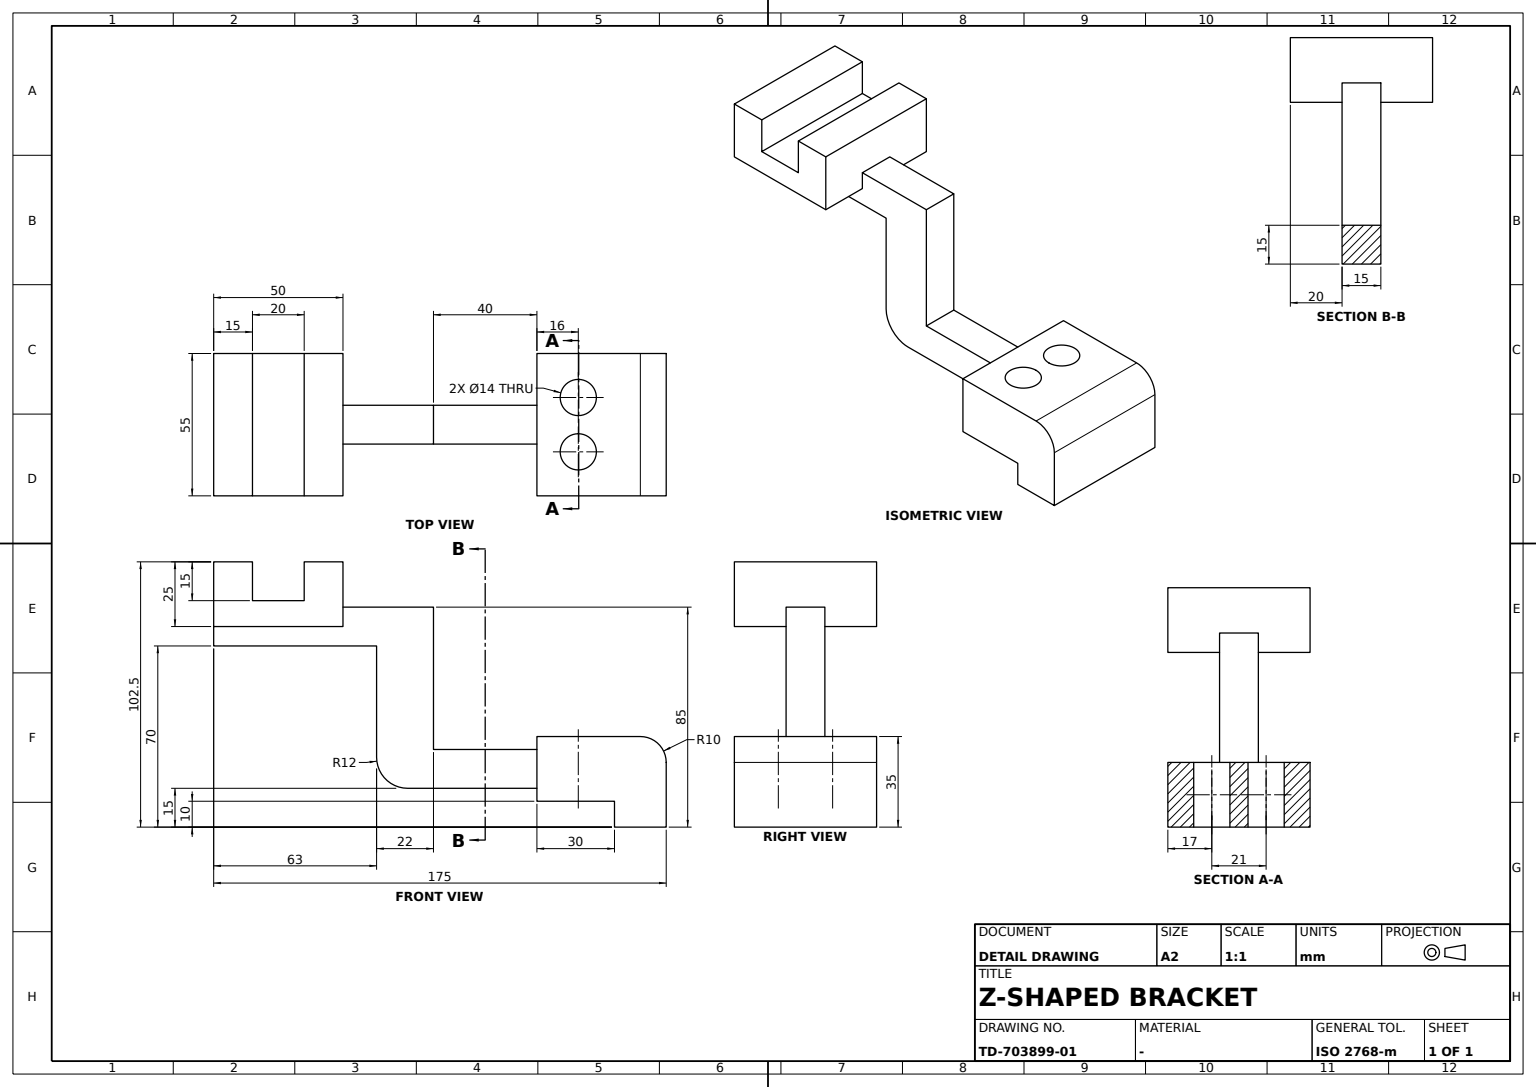
ISO-10303-21;
HEADER;
FILE_DESCRIPTION((''),'2;1');
FILE_NAME('','',(''),(''),'','','');
FILE_SCHEMA(('AUTOMOTIVE_DESIGN'));
ENDSEC;
DATA;
#1=APPLICATION_CONTEXT('');
#2=PRODUCT_CONTEXT('',#1,'mechanical');
#3=PRODUCT('','','',(#2));
#4=PRODUCT_DEFINITION_FORMATION('','',#3);
#5=PRODUCT_DEFINITION_CONTEXT('',#1,'design');
#6=PRODUCT_DEFINITION('','',#4,#5);
#7=PRODUCT_DEFINITION_SHAPE('','',#6);
#8=(LENGTH_UNIT()NAMED_UNIT(*)SI_UNIT(.MILLI.,.METRE.));
#9=(NAMED_UNIT(*)PLANE_ANGLE_UNIT()SI_UNIT($,.RADIAN.));
#10=(NAMED_UNIT(*)SI_UNIT($,.STERADIAN.)SOLID_ANGLE_UNIT());
#11=UNCERTAINTY_MEASURE_WITH_UNIT(LENGTH_MEASURE(0.005),#8,'distance_accuracy_value','');
#12=(GEOMETRIC_REPRESENTATION_CONTEXT(3)GLOBAL_UNCERTAINTY_ASSIGNED_CONTEXT((#11))GLOBAL_UNIT_ASSIGNED_CONTEXT((#8,#9,#10))REPRESENTATION_CONTEXT('',''));
#13=CARTESIAN_POINT('',(-17.5,78.,20.));
#14=VERTEX_POINT('',#13);
#15=CARTESIAN_POINT('',(-10.5,78.,20.));
#16=DIRECTION('',(0.,0.,-1.));
#17=DIRECTION('',(-1.,0.,0.));
#18=AXIS2_PLACEMENT_3D('',#15,#16,#17);
#19=CIRCLE('',#18,7.);
#20=EDGE_CURVE('',#14,#14,#19,.F.);
#21=ORIENTED_EDGE('',*,*,#20,.F.);
#22=EDGE_LOOP('',(#21));
#23=FACE_BOUND('',#22,.T.);
#24=CARTESIAN_POINT('',(3.5,78.,20.));
#25=VERTEX_POINT('',#24);
#26=CARTESIAN_POINT('',(10.5,78.,20.));
#27=AXIS2_PLACEMENT_3D('',#26,#16,#17);
#28=CIRCLE('',#27,7.);
#29=EDGE_CURVE('',#25,#25,#28,.F.);
#30=ORIENTED_EDGE('',*,*,#29,.F.);
#31=EDGE_LOOP('',(#30));
#32=FACE_BOUND('',#31,.T.);
#33=CARTESIAN_POINT('',(-27.5,62.,20.));
#34=VERTEX_POINT('',#33);
#35=CARTESIAN_POINT('',(27.5,62.,20.));
#36=VERTEX_POINT('',#35);
#37=CARTESIAN_POINT('',(0.,62.,20.));
#38=DIRECTION('',(1.,0.,0.));
#39=VECTOR('',#38,1000.);
#40=LINE('',#37,#39);
#41=EDGE_CURVE('',#34,#36,#40,.T.);
#42=ORIENTED_EDGE('',*,*,#41,.T.);
#43=CARTESIAN_POINT('',(27.5,102.,20.));
#44=VERTEX_POINT('',#43);
#45=CARTESIAN_POINT('',(27.5,0.,20.));
#46=DIRECTION('',(0.,1.,0.));
#47=VECTOR('',#46,1000.);
#48=LINE('',#45,#47);
#49=EDGE_CURVE('',#36,#44,#48,.T.);
#50=ORIENTED_EDGE('',*,*,#49,.T.);
#51=CARTESIAN_POINT('',(-27.5,102.,20.));
#52=VERTEX_POINT('',#51);
#53=CARTESIAN_POINT('',(0.,102.,20.));
#54=LINE('',#53,#39);
#55=EDGE_CURVE('',#52,#44,#54,.T.);
#56=ORIENTED_EDGE('',*,*,#55,.F.);
#57=CARTESIAN_POINT('',(-27.5,0.,20.));
#58=LINE('',#57,#47);
#59=EDGE_CURVE('',#34,#52,#58,.T.);
#60=ORIENTED_EDGE('',*,*,#59,.F.);
#61=EDGE_LOOP('',(#42,#50,#56,#60));
#62=FACE_BOUND('',#61,.T.);
#63=AXIS2_PLACEMENT_3D('',#37,#16,#46);
#64=PLANE('',#63);
#65=ADVANCED_FACE('',(#23,#32,#62),#64,.F.);
#66=CARTESIAN_POINT('',(-27.5,112.,10.));
#67=VERTEX_POINT('',#66);
#68=CARTESIAN_POINT('',(27.5,112.,10.));
#69=VERTEX_POINT('',#68);
#70=CARTESIAN_POINT('',(0.,112.,10.));
#71=LINE('',#70,#39);
#72=EDGE_CURVE('',#67,#69,#71,.T.);
#73=ORIENTED_EDGE('',*,*,#72,.F.);
#74=CARTESIAN_POINT('',(-27.5,102.,10.));
#75=AXIS2_PLACEMENT_3D('',#74,#38,#16);
#76=CIRCLE('',#75,10.);
#77=EDGE_CURVE('',#67,#52,#76,.T.);
#78=ORIENTED_EDGE('',*,*,#77,.T.);
#79=ORIENTED_EDGE('',*,*,#55,.T.);
#80=CARTESIAN_POINT('',(27.5,102.,10.));
#81=AXIS2_PLACEMENT_3D('',#80,#38,#16);
#82=CIRCLE('',#81,10.);
#83=EDGE_CURVE('',#69,#44,#82,.T.);
#84=ORIENTED_EDGE('',*,*,#83,.F.);
#85=EDGE_LOOP('',(#73,#78,#79,#84));
#86=FACE_BOUND('',#85,.T.);
#87=CARTESIAN_POINT('',(0.,102.,10.));
#88=DIRECTION('',(0.,0.,1.));
#89=AXIS2_PLACEMENT_3D('',#87,#38,#88);
#90=CYLINDRICAL_SURFACE('',#89,10.);
#91=ADVANCED_FACE('',(#86),#90,.T.);
#92=CARTESIAN_POINT('',(-27.5,62.,-5.));
#93=VERTEX_POINT('',#92);
#94=CARTESIAN_POINT('',(27.5,62.,-5.));
#95=VERTEX_POINT('',#94);
#96=CARTESIAN_POINT('',(0.,62.,-5.));
#97=LINE('',#96,#39);
#98=EDGE_CURVE('',#93,#95,#97,.T.);
#99=ORIENTED_EDGE('',*,*,#98,.F.);
#100=CARTESIAN_POINT('',(-27.5,92.,-5.));
#101=VERTEX_POINT('',#100);
#102=CARTESIAN_POINT('',(-27.5,0.,-5.));
#103=DIRECTION('',(0.,-1.,0.));
#104=VECTOR('',#103,1000.);
#105=LINE('',#102,#104);
#106=EDGE_CURVE('',#101,#93,#105,.T.);
#107=ORIENTED_EDGE('',*,*,#106,.F.);
#108=CARTESIAN_POINT('',(27.5,92.,-5.));
#109=VERTEX_POINT('',#108);
#110=CARTESIAN_POINT('',(0.,92.,-5.));
#111=LINE('',#110,#39);
#112=EDGE_CURVE('',#101,#109,#111,.T.);
#113=ORIENTED_EDGE('',*,*,#112,.T.);
#114=CARTESIAN_POINT('',(27.5,0.,-5.));
#115=LINE('',#114,#104);
#116=EDGE_CURVE('',#109,#95,#115,.T.);
#117=ORIENTED_EDGE('',*,*,#116,.T.);
#118=EDGE_LOOP('',(#99,#107,#113,#117));
#119=FACE_BOUND('',#118,.T.);
#120=CARTESIAN_POINT('',(-3.5,78.,-5.));
#121=VERTEX_POINT('',#120);
#122=CARTESIAN_POINT('',(-10.5,78.,-5.));
#123=AXIS2_PLACEMENT_3D('',#122,#88,#38);
#124=CIRCLE('',#123,7.);
#125=EDGE_CURVE('',#121,#121,#124,.T.);
#126=ORIENTED_EDGE('',*,*,#125,.T.);
#127=EDGE_LOOP('',(#126));
#128=FACE_BOUND('',#127,.T.);
#129=CARTESIAN_POINT('',(17.5,78.,-5.));
#130=VERTEX_POINT('',#129);
#131=CARTESIAN_POINT('',(10.5,78.,-5.));
#132=AXIS2_PLACEMENT_3D('',#131,#88,#38);
#133=CIRCLE('',#132,7.);
#134=EDGE_CURVE('',#130,#130,#133,.T.);
#135=ORIENTED_EDGE('',*,*,#134,.T.);
#136=EDGE_LOOP('',(#135));
#137=FACE_BOUND('',#136,.T.);
#138=AXIS2_PLACEMENT_3D('',#110,#88,#103);
#139=PLANE('',#138);
#140=ADVANCED_FACE('',(#119,#128,#137),#139,.F.);
#141=CARTESIAN_POINT('',(-27.5,-28.,72.5));
#142=VERTEX_POINT('',#141);
#143=CARTESIAN_POINT('',(27.5,-28.,72.5));
#144=VERTEX_POINT('',#143);
#145=CARTESIAN_POINT('',(0.,-28.,72.5));
#146=LINE('',#145,#39);
#147=EDGE_CURVE('',#142,#144,#146,.T.);
#148=ORIENTED_EDGE('',*,*,#147,.T.);
#149=CARTESIAN_POINT('',(27.5,-28.,87.5));
#150=VERTEX_POINT('',#149);
#151=CARTESIAN_POINT('',(27.5,-28.,0.));
#152=VECTOR('',#88,1000.);
#153=LINE('',#151,#152);
#154=EDGE_CURVE('',#144,#150,#153,.T.);
#155=ORIENTED_EDGE('',*,*,#154,.T.);
#156=CARTESIAN_POINT('',(-27.5,-28.,87.5));
#157=VERTEX_POINT('',#156);
#158=CARTESIAN_POINT('',(0.,-28.,87.5));
#159=LINE('',#158,#39);
#160=EDGE_CURVE('',#157,#150,#159,.T.);
#161=ORIENTED_EDGE('',*,*,#160,.F.);
#162=CARTESIAN_POINT('',(-27.5,-28.,0.));
#163=LINE('',#162,#152);
#164=EDGE_CURVE('',#142,#157,#163,.T.);
#165=ORIENTED_EDGE('',*,*,#164,.F.);
#166=EDGE_LOOP('',(#148,#155,#161,#165));
#167=FACE_BOUND('',#166,.T.);
#168=AXIS2_PLACEMENT_3D('',#145,#46,#88);
#169=PLANE('',#168);
#170=ADVANCED_FACE('',(#167),#169,.F.);
#171=CARTESIAN_POINT('',(7.5,22.,15.));
#172=VERTEX_POINT('',#171);
#173=CARTESIAN_POINT('',(7.5,62.,15.));
#174=VERTEX_POINT('',#173);
#175=CARTESIAN_POINT('',(7.5,0.,15.));
#176=LINE('',#175,#47);
#177=EDGE_CURVE('',#172,#174,#176,.T.);
#178=ORIENTED_EDGE('',*,*,#177,.T.);
#179=CARTESIAN_POINT('',(-7.5,62.,15.));
#180=VERTEX_POINT('',#179);
#181=CARTESIAN_POINT('',(0.,62.,15.));
#182=LINE('',#181,#39);
#183=EDGE_CURVE('',#180,#174,#182,.T.);
#184=ORIENTED_EDGE('',*,*,#183,.F.);
#185=CARTESIAN_POINT('',(-7.5,22.,15.));
#186=VERTEX_POINT('',#185);
#187=CARTESIAN_POINT('',(-7.5,0.,15.));
#188=LINE('',#187,#47);
#189=EDGE_CURVE('',#186,#180,#188,.T.);
#190=ORIENTED_EDGE('',*,*,#189,.F.);
#191=CARTESIAN_POINT('',(0.,22.,15.));
#192=LINE('',#191,#39);
#193=EDGE_CURVE('',#186,#172,#192,.T.);
#194=ORIENTED_EDGE('',*,*,#193,.T.);
#195=EDGE_LOOP('',(#178,#184,#190,#194));
#196=FACE_BOUND('',#195,.T.);
#197=AXIS2_PLACEMENT_3D('',#191,#16,#46);
#198=PLANE('',#197);
#199=ADVANCED_FACE('',(#196),#198,.F.);
#200=ORIENTED_EDGE('',*,*,#106,.T.);
#201=CARTESIAN_POINT('',(-27.5,62.,15.));
#202=LINE('',#201,#152);
#203=EDGE_CURVE('',#93,#34,#202,.T.);
#204=ORIENTED_EDGE('',*,*,#203,.T.);
#205=ORIENTED_EDGE('',*,*,#59,.T.);
#206=ORIENTED_EDGE('',*,*,#77,.F.);
#207=CARTESIAN_POINT('',(-27.5,112.,-15.));
#208=VERTEX_POINT('',#207);
#209=CARTESIAN_POINT('',(-27.5,112.,0.));
#210=VECTOR('',#16,1000.);
#211=LINE('',#209,#210);
#212=EDGE_CURVE('',#67,#208,#211,.T.);
#213=ORIENTED_EDGE('',*,*,#212,.T.);
#214=CARTESIAN_POINT('',(-27.5,92.,-15.));
#215=VERTEX_POINT('',#214);
#216=CARTESIAN_POINT('',(-27.5,0.,-15.));
#217=LINE('',#216,#104);
#218=EDGE_CURVE('',#208,#215,#217,.T.);
#219=ORIENTED_EDGE('',*,*,#218,.T.);
#220=CARTESIAN_POINT('',(-27.5,92.,0.));
#221=LINE('',#220,#152);
#222=EDGE_CURVE('',#215,#101,#221,.T.);
#223=ORIENTED_EDGE('',*,*,#222,.T.);
#224=EDGE_LOOP('',(#200,#204,#205,#206,#213,#219,#223));
#225=FACE_BOUND('',#224,.T.);
#226=CARTESIAN_POINT('',(-27.5,0.,0.));
#227=AXIS2_PLACEMENT_3D('',#226,#38,#46);
#228=PLANE('',#227);
#229=ADVANCED_FACE('',(#225),#228,.F.);
#230=CARTESIAN_POINT('',(-7.5,0.,55.));
#231=VERTEX_POINT('',#230);
#232=CARTESIAN_POINT('',(-7.5,-63.,55.));
#233=VERTEX_POINT('',#232);
#234=LINE('',#232,#104);
#235=EDGE_CURVE('',#231,#233,#234,.T.);
#236=ORIENTED_EDGE('',*,*,#235,.T.);
#237=CARTESIAN_POINT('',(-7.5,-63.,62.5));
#238=VERTEX_POINT('',#237);
#239=CARTESIAN_POINT('',(-7.5,-63.,0.));
#240=LINE('',#239,#152);
#241=EDGE_CURVE('',#233,#238,#240,.T.);
#242=ORIENTED_EDGE('',*,*,#241,.T.);
#243=CARTESIAN_POINT('',(-7.5,-13.,62.5));
#244=VERTEX_POINT('',#243);
#245=CARTESIAN_POINT('',(-7.5,0.,62.5));
#246=LINE('',#245,#104);
#247=EDGE_CURVE('',#244,#238,#246,.T.);
#248=ORIENTED_EDGE('',*,*,#247,.F.);
#249=CARTESIAN_POINT('',(-7.5,-13.,70.));
#250=VERTEX_POINT('',#249);
#251=CARTESIAN_POINT('',(-7.5,-13.,0.));
#252=LINE('',#251,#152);
#253=EDGE_CURVE('',#244,#250,#252,.T.);
#254=ORIENTED_EDGE('',*,*,#253,.T.);
#255=CARTESIAN_POINT('',(-7.5,22.,70.));
#256=VERTEX_POINT('',#255);
#257=CARTESIAN_POINT('',(-7.5,0.,70.));
#258=LINE('',#257,#47);
#259=EDGE_CURVE('',#250,#256,#258,.T.);
#260=ORIENTED_EDGE('',*,*,#259,.T.);
#261=CARTESIAN_POINT('',(-7.5,22.,0.));
#262=LINE('',#261,#210);
#263=EDGE_CURVE('',#256,#186,#262,.T.);
#264=ORIENTED_EDGE('',*,*,#263,.T.);
#265=ORIENTED_EDGE('',*,*,#189,.T.);
#266=CARTESIAN_POINT('',(-7.5,62.,0.));
#267=VERTEX_POINT('',#266);
#268=LINE('',#266,#210);
#269=EDGE_CURVE('',#180,#267,#268,.T.);
#270=ORIENTED_EDGE('',*,*,#269,.T.);
#271=CARTESIAN_POINT('',(-7.5,12.,0.));
#272=VERTEX_POINT('',#271);
#273=CARTESIAN_POINT('',(-7.5,0.,0.));
#274=LINE('',#273,#104);
#275=EDGE_CURVE('',#267,#272,#274,.T.);
#276=ORIENTED_EDGE('',*,*,#275,.T.);
#277=CARTESIAN_POINT('',(-7.5,0.,12.));
#278=VERTEX_POINT('',#277);
#279=CARTESIAN_POINT('',(-7.5,12.,12.));
#280=AXIS2_PLACEMENT_3D('',#279,#38,#16);
#281=CIRCLE('',#280,12.);
#282=EDGE_CURVE('',#278,#272,#281,.T.);
#283=ORIENTED_EDGE('',*,*,#282,.F.);
#284=LINE('',#273,#152);
#285=EDGE_CURVE('',#278,#231,#284,.T.);
#286=ORIENTED_EDGE('',*,*,#285,.T.);
#287=EDGE_LOOP('',(#236,#242,#248,#254,#260,#264,#265,#270,#276,#283,#286));
#288=FACE_BOUND('',#287,.T.);
#289=AXIS2_PLACEMENT_3D('',#273,#38,#46);
#290=PLANE('',#289);
#291=ADVANCED_FACE('',(#288),#290,.F.);
#292=CARTESIAN_POINT('',(27.5,-13.,62.5));
#293=VERTEX_POINT('',#292);
#294=CARTESIAN_POINT('',(27.5,-63.,62.5));
#295=VERTEX_POINT('',#294);
#296=CARTESIAN_POINT('',(27.5,0.,62.5));
#297=LINE('',#296,#104);
#298=EDGE_CURVE('',#293,#295,#297,.T.);
#299=ORIENTED_EDGE('',*,*,#298,.F.);
#300=CARTESIAN_POINT('',(27.5,-13.,87.5));
#301=VERTEX_POINT('',#300);
#302=LINE('',#292,#210);
#303=EDGE_CURVE('',#301,#293,#302,.T.);
#304=ORIENTED_EDGE('',*,*,#303,.F.);
#305=CARTESIAN_POINT('',(27.5,0.,87.5));
#306=LINE('',#305,#47);
#307=EDGE_CURVE('',#150,#301,#306,.T.);
#308=ORIENTED_EDGE('',*,*,#307,.F.);
#309=ORIENTED_EDGE('',*,*,#154,.F.);
#310=CARTESIAN_POINT('',(27.5,-48.,72.5));
#311=VERTEX_POINT('',#310);
#312=CARTESIAN_POINT('',(27.5,0.,72.5));
#313=LINE('',#312,#47);
#314=EDGE_CURVE('',#311,#144,#313,.T.);
#315=ORIENTED_EDGE('',*,*,#314,.F.);
#316=CARTESIAN_POINT('',(27.5,-48.,87.5));
#317=VERTEX_POINT('',#316);
#318=CARTESIAN_POINT('',(27.5,-48.,0.));
#319=LINE('',#318,#210);
#320=EDGE_CURVE('',#317,#311,#319,.T.);
#321=ORIENTED_EDGE('',*,*,#320,.F.);
#322=CARTESIAN_POINT('',(27.5,-63.,87.5));
#323=VERTEX_POINT('',#322);
#324=EDGE_CURVE('',#323,#317,#306,.T.);
#325=ORIENTED_EDGE('',*,*,#324,.F.);
#326=CARTESIAN_POINT('',(27.5,-63.,0.));
#327=LINE('',#326,#152);
#328=EDGE_CURVE('',#295,#323,#327,.T.);
#329=ORIENTED_EDGE('',*,*,#328,.F.);
#330=EDGE_LOOP('',(#299,#304,#308,#309,#315,#321,#325,#329));
#331=FACE_BOUND('',#330,.T.);
#332=CARTESIAN_POINT('',(27.5,0.,0.));
#333=AXIS2_PLACEMENT_3D('',#332,#38,#46);
#334=PLANE('',#333);
#335=ADVANCED_FACE('',(#331),#334,.T.);
#336=CARTESIAN_POINT('',(-27.5,-63.,87.5));
#337=VERTEX_POINT('',#336);
#338=CARTESIAN_POINT('',(0.,-63.,87.5));
#339=LINE('',#338,#39);
#340=EDGE_CURVE('',#337,#323,#339,.T.);
#341=ORIENTED_EDGE('',*,*,#340,.T.);
#342=ORIENTED_EDGE('',*,*,#324,.T.);
#343=CARTESIAN_POINT('',(-27.5,-48.,87.5));
#344=VERTEX_POINT('',#343);
#345=CARTESIAN_POINT('',(0.,-48.,87.5));
#346=LINE('',#345,#39);
#347=EDGE_CURVE('',#344,#317,#346,.T.);
#348=ORIENTED_EDGE('',*,*,#347,.F.);
#349=CARTESIAN_POINT('',(-27.5,0.,87.5));
#350=LINE('',#349,#47);
#351=EDGE_CURVE('',#337,#344,#350,.T.);
#352=ORIENTED_EDGE('',*,*,#351,.F.);
#353=EDGE_LOOP('',(#341,#342,#348,#352));
#354=FACE_BOUND('',#353,.T.);
#355=AXIS2_PLACEMENT_3D('',#158,#16,#46);
#356=PLANE('',#355);
#357=ADVANCED_FACE('',(#354),#356,.F.);
#358=ORIENTED_EDGE('',*,*,#112,.F.);
#359=ORIENTED_EDGE('',*,*,#222,.F.);
#360=CARTESIAN_POINT('',(27.5,92.,-15.));
#361=VERTEX_POINT('',#360);
#362=CARTESIAN_POINT('',(0.,92.,-15.));
#363=LINE('',#362,#39);
#364=EDGE_CURVE('',#215,#361,#363,.T.);
#365=ORIENTED_EDGE('',*,*,#364,.T.);
#366=CARTESIAN_POINT('',(27.5,92.,0.));
#367=LINE('',#366,#152);
#368=EDGE_CURVE('',#361,#109,#367,.T.);
#369=ORIENTED_EDGE('',*,*,#368,.T.);
#370=EDGE_LOOP('',(#358,#359,#365,#369));
#371=FACE_BOUND('',#370,.T.);
#372=AXIS2_PLACEMENT_3D('',#362,#46,#88);
#373=PLANE('',#372);
#374=ADVANCED_FACE('',(#371),#373,.F.);
#375=CARTESIAN_POINT('',(27.5,112.,-15.));
#376=VERTEX_POINT('',#375);
#377=CARTESIAN_POINT('',(0.,112.,-15.));
#378=LINE('',#377,#39);
#379=EDGE_CURVE('',#208,#376,#378,.T.);
#380=ORIENTED_EDGE('',*,*,#379,.F.);
#381=ORIENTED_EDGE('',*,*,#212,.F.);
#382=ORIENTED_EDGE('',*,*,#72,.T.);
#383=CARTESIAN_POINT('',(27.5,112.,0.));
#384=LINE('',#383,#210);
#385=EDGE_CURVE('',#69,#376,#384,.T.);
#386=ORIENTED_EDGE('',*,*,#385,.T.);
#387=EDGE_LOOP('',(#380,#381,#382,#386));
#388=FACE_BOUND('',#387,.T.);
#389=CARTESIAN_POINT('',(0.,112.,20.));
#390=AXIS2_PLACEMENT_3D('',#389,#103,#16);
#391=PLANE('',#390);
#392=ADVANCED_FACE('',(#388),#391,.F.);
#393=CARTESIAN_POINT('',(-27.5,-13.,62.5));
#394=VERTEX_POINT('',#393);
#395=CARTESIAN_POINT('',(-27.5,-63.,62.5));
#396=VERTEX_POINT('',#395);
#397=CARTESIAN_POINT('',(-27.5,0.,62.5));
#398=LINE('',#397,#104);
#399=EDGE_CURVE('',#394,#396,#398,.T.);
#400=ORIENTED_EDGE('',*,*,#399,.T.);
#401=CARTESIAN_POINT('',(-27.5,-63.,0.));
#402=LINE('',#401,#152);
#403=EDGE_CURVE('',#396,#337,#402,.T.);
#404=ORIENTED_EDGE('',*,*,#403,.T.);
#405=ORIENTED_EDGE('',*,*,#351,.T.);
#406=CARTESIAN_POINT('',(-27.5,-48.,72.5));
#407=VERTEX_POINT('',#406);
#408=CARTESIAN_POINT('',(-27.5,-48.,0.));
#409=LINE('',#408,#210);
#410=EDGE_CURVE('',#344,#407,#409,.T.);
#411=ORIENTED_EDGE('',*,*,#410,.T.);
#412=CARTESIAN_POINT('',(-27.5,0.,72.5));
#413=LINE('',#412,#47);
#414=EDGE_CURVE('',#407,#142,#413,.T.);
#415=ORIENTED_EDGE('',*,*,#414,.T.);
#416=ORIENTED_EDGE('',*,*,#164,.T.);
#417=CARTESIAN_POINT('',(-27.5,-13.,87.5));
#418=VERTEX_POINT('',#417);
#419=EDGE_CURVE('',#157,#418,#350,.T.);
#420=ORIENTED_EDGE('',*,*,#419,.T.);
#421=LINE('',#393,#210);
#422=EDGE_CURVE('',#418,#394,#421,.T.);
#423=ORIENTED_EDGE('',*,*,#422,.T.);
#424=EDGE_LOOP('',(#400,#404,#405,#411,#415,#416,#420,#423));
#425=FACE_BOUND('',#424,.T.);
#426=ADVANCED_FACE('',(#425),#228,.F.);
#427=ORIENTED_EDGE('',*,*,#241,.F.);
#428=CARTESIAN_POINT('',(7.5,-63.,55.));
#429=VERTEX_POINT('',#428);
#430=CARTESIAN_POINT('',(0.,-63.,55.));
#431=LINE('',#430,#39);
#432=EDGE_CURVE('',#233,#429,#431,.T.);
#433=ORIENTED_EDGE('',*,*,#432,.T.);
#434=CARTESIAN_POINT('',(7.5,-63.,62.5));
#435=VERTEX_POINT('',#434);
#436=CARTESIAN_POINT('',(7.5,-63.,0.));
#437=LINE('',#436,#152);
#438=EDGE_CURVE('',#429,#435,#437,.T.);
#439=ORIENTED_EDGE('',*,*,#438,.T.);
#440=CARTESIAN_POINT('',(0.,-63.,62.5));
#441=LINE('',#440,#39);
#442=EDGE_CURVE('',#435,#295,#441,.T.);
#443=ORIENTED_EDGE('',*,*,#442,.T.);
#444=ORIENTED_EDGE('',*,*,#328,.T.);
#445=ORIENTED_EDGE('',*,*,#340,.F.);
#446=ORIENTED_EDGE('',*,*,#403,.F.);
#447=EDGE_CURVE('',#396,#238,#441,.T.);
#448=ORIENTED_EDGE('',*,*,#447,.T.);
#449=EDGE_LOOP('',(#427,#433,#439,#443,#444,#445,#446,#448));
#450=FACE_BOUND('',#449,.T.);
#451=AXIS2_PLACEMENT_3D('',#430,#46,#88);
#452=PLANE('',#451);
#453=ADVANCED_FACE('',(#450),#452,.F.);
#454=ORIENTED_EDGE('',*,*,#379,.T.);
#455=CARTESIAN_POINT('',(27.5,0.,-15.));
#456=LINE('',#455,#104);
#457=EDGE_CURVE('',#376,#361,#456,.T.);
#458=ORIENTED_EDGE('',*,*,#457,.T.);
#459=ORIENTED_EDGE('',*,*,#364,.F.);
#460=ORIENTED_EDGE('',*,*,#218,.F.);
#461=EDGE_LOOP('',(#454,#458,#459,#460));
#462=FACE_BOUND('',#461,.T.);
#463=AXIS2_PLACEMENT_3D('',#377,#88,#103);
#464=PLANE('',#463);
#465=ADVANCED_FACE('',(#462),#464,.F.);
#466=CARTESIAN_POINT('',(7.5,0.,55.));
#467=VERTEX_POINT('',#466);
#468=CARTESIAN_POINT('',(0.,0.,55.));
#469=LINE('',#468,#39);
#470=EDGE_CURVE('',#231,#467,#469,.T.);
#471=ORIENTED_EDGE('',*,*,#470,.T.);
#472=LINE('',#466,#47);
#473=EDGE_CURVE('',#429,#467,#472,.T.);
#474=ORIENTED_EDGE('',*,*,#473,.F.);
#475=ORIENTED_EDGE('',*,*,#432,.F.);
#476=ORIENTED_EDGE('',*,*,#235,.F.);
#477=EDGE_LOOP('',(#471,#474,#475,#476));
#478=FACE_BOUND('',#477,.T.);
#479=AXIS2_PLACEMENT_3D('',#430,#16,#46);
#480=PLANE('',#479);
#481=ADVANCED_FACE('',(#478),#480,.T.);
#482=ORIENTED_EDGE('',*,*,#457,.F.);
#483=ORIENTED_EDGE('',*,*,#385,.F.);
#484=ORIENTED_EDGE('',*,*,#83,.T.);
#485=ORIENTED_EDGE('',*,*,#49,.F.);
#486=CARTESIAN_POINT('',(27.5,62.,15.));
#487=LINE('',#486,#152);
#488=EDGE_CURVE('',#95,#36,#487,.T.);
#489=ORIENTED_EDGE('',*,*,#488,.F.);
#490=ORIENTED_EDGE('',*,*,#116,.F.);
#491=ORIENTED_EDGE('',*,*,#368,.F.);
#492=EDGE_LOOP('',(#482,#483,#484,#485,#489,#490,#491));
#493=FACE_BOUND('',#492,.T.);
#494=ADVANCED_FACE('',(#493),#334,.T.);
#495=ORIENTED_EDGE('',*,*,#447,.F.);
#496=ORIENTED_EDGE('',*,*,#399,.F.);
#497=CARTESIAN_POINT('',(0.,-13.,62.5));
#498=LINE('',#497,#39);
#499=EDGE_CURVE('',#394,#244,#498,.T.);
#500=ORIENTED_EDGE('',*,*,#499,.T.);
#501=ORIENTED_EDGE('',*,*,#247,.T.);
#502=EDGE_LOOP('',(#495,#496,#500,#501));
#503=FACE_BOUND('',#502,.T.);
#504=AXIS2_PLACEMENT_3D('',#497,#88,#103);
#505=PLANE('',#504);
#506=ADVANCED_FACE('',(#503),#505,.F.);
#507=ORIENTED_EDGE('',*,*,#160,.T.);
#508=ORIENTED_EDGE('',*,*,#307,.T.);
#509=CARTESIAN_POINT('',(0.,-13.,87.5));
#510=LINE('',#509,#39);
#511=EDGE_CURVE('',#418,#301,#510,.T.);
#512=ORIENTED_EDGE('',*,*,#511,.F.);
#513=ORIENTED_EDGE('',*,*,#419,.F.);
#514=EDGE_LOOP('',(#507,#508,#512,#513));
#515=FACE_BOUND('',#514,.T.);
#516=ADVANCED_FACE('',(#515),#356,.F.);
#517=ORIENTED_EDGE('',*,*,#147,.F.);
#518=ORIENTED_EDGE('',*,*,#414,.F.);
#519=CARTESIAN_POINT('',(0.,-48.,72.5));
#520=LINE('',#519,#39);
#521=EDGE_CURVE('',#407,#311,#520,.T.);
#522=ORIENTED_EDGE('',*,*,#521,.T.);
#523=ORIENTED_EDGE('',*,*,#314,.T.);
#524=EDGE_LOOP('',(#517,#518,#522,#523));
#525=FACE_BOUND('',#524,.T.);
#526=AXIS2_PLACEMENT_3D('',#519,#16,#46);
#527=PLANE('',#526);
#528=ADVANCED_FACE('',(#525),#527,.F.);
#529=ORIENTED_EDGE('',*,*,#470,.F.);
#530=ORIENTED_EDGE('',*,*,#285,.F.);
#531=CARTESIAN_POINT('',(7.5,0.,12.));
#532=VERTEX_POINT('',#531);
#533=CARTESIAN_POINT('',(0.,0.,12.));
#534=LINE('',#533,#39);
#535=EDGE_CURVE('',#278,#532,#534,.T.);
#536=ORIENTED_EDGE('',*,*,#535,.T.);
#537=CARTESIAN_POINT('',(7.5,0.,0.));
#538=LINE('',#537,#152);
#539=EDGE_CURVE('',#532,#467,#538,.T.);
#540=ORIENTED_EDGE('',*,*,#539,.T.);
#541=EDGE_LOOP('',(#529,#530,#536,#540));
#542=FACE_BOUND('',#541,.T.);
#543=CARTESIAN_POINT('',(0.,0.,0.));
#544=AXIS2_PLACEMENT_3D('',#543,#46,#88);
#545=PLANE('',#544);
#546=ADVANCED_FACE('',(#542),#545,.F.);
#547=CARTESIAN_POINT('',(7.5,-13.,70.));
#548=VERTEX_POINT('',#547);
#549=CARTESIAN_POINT('',(0.,-13.,70.));
#550=LINE('',#549,#39);
#551=EDGE_CURVE('',#250,#548,#550,.T.);
#552=ORIENTED_EDGE('',*,*,#551,.T.);
#553=CARTESIAN_POINT('',(7.5,22.,70.));
#554=VERTEX_POINT('',#553);
#555=CARTESIAN_POINT('',(7.5,0.,70.));
#556=LINE('',#555,#47);
#557=EDGE_CURVE('',#548,#554,#556,.T.);
#558=ORIENTED_EDGE('',*,*,#557,.T.);
#559=CARTESIAN_POINT('',(0.,22.,70.));
#560=LINE('',#559,#39);
#561=EDGE_CURVE('',#256,#554,#560,.T.);
#562=ORIENTED_EDGE('',*,*,#561,.F.);
#563=ORIENTED_EDGE('',*,*,#259,.F.);
#564=EDGE_LOOP('',(#552,#558,#562,#563));
#565=FACE_BOUND('',#564,.T.);
#566=AXIS2_PLACEMENT_3D('',#549,#16,#46);
#567=PLANE('',#566);
#568=ADVANCED_FACE('',(#565),#567,.F.);
#569=CARTESIAN_POINT('',(7.5,-13.,62.5));
#570=VERTEX_POINT('',#569);
#571=CARTESIAN_POINT('',(7.5,0.,62.5));
#572=LINE('',#571,#104);
#573=EDGE_CURVE('',#570,#435,#572,.T.);
#574=ORIENTED_EDGE('',*,*,#573,.F.);
#575=EDGE_CURVE('',#570,#293,#498,.T.);
#576=ORIENTED_EDGE('',*,*,#575,.T.);
#577=ORIENTED_EDGE('',*,*,#298,.T.);
#578=ORIENTED_EDGE('',*,*,#442,.F.);
#579=EDGE_LOOP('',(#574,#576,#577,#578));
#580=FACE_BOUND('',#579,.T.);
#581=ADVANCED_FACE('',(#580),#505,.F.);
#582=ORIENTED_EDGE('',*,*,#263,.F.);
#583=ORIENTED_EDGE('',*,*,#561,.T.);
#584=CARTESIAN_POINT('',(7.5,22.,0.));
#585=LINE('',#584,#210);
#586=EDGE_CURVE('',#554,#172,#585,.T.);
#587=ORIENTED_EDGE('',*,*,#586,.T.);
#588=ORIENTED_EDGE('',*,*,#193,.F.);
#589=EDGE_LOOP('',(#582,#583,#587,#588));
#590=FACE_BOUND('',#589,.T.);
#591=AXIS2_PLACEMENT_3D('',#559,#103,#16);
#592=PLANE('',#591);
#593=ADVANCED_FACE('',(#590),#592,.F.);
#594=ORIENTED_EDGE('',*,*,#29,.T.);
#595=EDGE_LOOP('',(#594));
#596=FACE_BOUND('',#595,.T.);
#597=ORIENTED_EDGE('',*,*,#134,.F.);
#598=EDGE_LOOP('',(#597));
#599=FACE_BOUND('',#598,.T.);
#600=CARTESIAN_POINT('',(10.5,78.,1.84));
#601=AXIS2_PLACEMENT_3D('',#600,#88,#38);
#602=CYLINDRICAL_SURFACE('',#601,7.);
#603=ADVANCED_FACE('',(#596,#599),#602,.F.);
#604=ORIENTED_EDGE('',*,*,#275,.F.);
#605=CARTESIAN_POINT('',(7.5,62.,0.));
#606=VERTEX_POINT('',#605);
#607=CARTESIAN_POINT('',(0.,62.,0.));
#608=LINE('',#607,#39);
#609=EDGE_CURVE('',#267,#606,#608,.T.);
#610=ORIENTED_EDGE('',*,*,#609,.T.);
#611=CARTESIAN_POINT('',(7.5,12.,0.));
#612=VERTEX_POINT('',#611);
#613=LINE('',#537,#104);
#614=EDGE_CURVE('',#606,#612,#613,.T.);
#615=ORIENTED_EDGE('',*,*,#614,.T.);
#616=CARTESIAN_POINT('',(0.,12.,0.));
#617=LINE('',#616,#39);
#618=EDGE_CURVE('',#272,#612,#617,.T.);
#619=ORIENTED_EDGE('',*,*,#618,.F.);
#620=EDGE_LOOP('',(#604,#610,#615,#619));
#621=FACE_BOUND('',#620,.T.);
#622=AXIS2_PLACEMENT_3D('',#607,#88,#103);
#623=PLANE('',#622);
#624=ADVANCED_FACE('',(#621),#623,.F.);
#625=ORIENTED_EDGE('',*,*,#573,.T.);
#626=ORIENTED_EDGE('',*,*,#438,.F.);
#627=ORIENTED_EDGE('',*,*,#473,.T.);
#628=ORIENTED_EDGE('',*,*,#539,.F.);
#629=CARTESIAN_POINT('',(7.5,12.,12.));
#630=AXIS2_PLACEMENT_3D('',#629,#38,#16);
#631=CIRCLE('',#630,12.);
#632=EDGE_CURVE('',#532,#612,#631,.T.);
#633=ORIENTED_EDGE('',*,*,#632,.T.);
#634=ORIENTED_EDGE('',*,*,#614,.F.);
#635=LINE('',#605,#210);
#636=EDGE_CURVE('',#174,#606,#635,.T.);
#637=ORIENTED_EDGE('',*,*,#636,.F.);
#638=ORIENTED_EDGE('',*,*,#177,.F.);
#639=ORIENTED_EDGE('',*,*,#586,.F.);
#640=ORIENTED_EDGE('',*,*,#557,.F.);
#641=CARTESIAN_POINT('',(7.5,-13.,0.));
#642=LINE('',#641,#152);
#643=EDGE_CURVE('',#570,#548,#642,.T.);
#644=ORIENTED_EDGE('',*,*,#643,.F.);
#645=EDGE_LOOP('',(#625,#626,#627,#628,#633,#634,#637,#638,#639,#640,#644));
#646=FACE_BOUND('',#645,.T.);
#647=AXIS2_PLACEMENT_3D('',#537,#38,#46);
#648=PLANE('',#647);
#649=ADVANCED_FACE('',(#646),#648,.T.);
#650=ORIENTED_EDGE('',*,*,#347,.T.);
#651=ORIENTED_EDGE('',*,*,#320,.T.);
#652=ORIENTED_EDGE('',*,*,#521,.F.);
#653=ORIENTED_EDGE('',*,*,#410,.F.);
#654=EDGE_LOOP('',(#650,#651,#652,#653));
#655=FACE_BOUND('',#654,.T.);
#656=AXIS2_PLACEMENT_3D('',#345,#103,#16);
#657=PLANE('',#656);
#658=ADVANCED_FACE('',(#655),#657,.F.);
#659=ORIENTED_EDGE('',*,*,#20,.T.);
#660=EDGE_LOOP('',(#659));
#661=FACE_BOUND('',#660,.T.);
#662=ORIENTED_EDGE('',*,*,#125,.F.);
#663=EDGE_LOOP('',(#662));
#664=FACE_BOUND('',#663,.T.);
#665=CARTESIAN_POINT('',(-10.5,78.,1.84));
#666=AXIS2_PLACEMENT_3D('',#665,#88,#38);
#667=CYLINDRICAL_SURFACE('',#666,7.);
#668=ADVANCED_FACE('',(#661,#664),#667,.F.);
#669=ORIENTED_EDGE('',*,*,#511,.T.);
#670=ORIENTED_EDGE('',*,*,#303,.T.);
#671=ORIENTED_EDGE('',*,*,#575,.F.);
#672=ORIENTED_EDGE('',*,*,#643,.T.);
#673=ORIENTED_EDGE('',*,*,#551,.F.);
#674=ORIENTED_EDGE('',*,*,#253,.F.);
#675=ORIENTED_EDGE('',*,*,#499,.F.);
#676=ORIENTED_EDGE('',*,*,#422,.F.);
#677=EDGE_LOOP('',(#669,#670,#671,#672,#673,#674,#675,#676));
#678=FACE_BOUND('',#677,.T.);
#679=AXIS2_PLACEMENT_3D('',#497,#46,#88);
#680=PLANE('',#679);
#681=ADVANCED_FACE('',(#678),#680,.T.);
#682=ORIENTED_EDGE('',*,*,#282,.T.);
#683=ORIENTED_EDGE('',*,*,#618,.T.);
#684=ORIENTED_EDGE('',*,*,#632,.F.);
#685=ORIENTED_EDGE('',*,*,#535,.F.);
#686=EDGE_LOOP('',(#682,#683,#684,#685));
#687=FACE_BOUND('',#686,.T.);
#688=CARTESIAN_POINT('',(0.,12.,12.));
#689=AXIS2_PLACEMENT_3D('',#688,#38,#16);
#690=CYLINDRICAL_SURFACE('',#689,12.);
#691=ADVANCED_FACE('',(#687),#690,.T.);
#692=ORIENTED_EDGE('',*,*,#203,.F.);
#693=ORIENTED_EDGE('',*,*,#98,.T.);
#694=ORIENTED_EDGE('',*,*,#488,.T.);
#695=ORIENTED_EDGE('',*,*,#41,.F.);
#696=EDGE_LOOP('',(#692,#693,#694,#695));
#697=FACE_BOUND('',#696,.T.);
#698=ORIENTED_EDGE('',*,*,#636,.T.);
#699=ORIENTED_EDGE('',*,*,#609,.F.);
#700=ORIENTED_EDGE('',*,*,#269,.F.);
#701=ORIENTED_EDGE('',*,*,#183,.T.);
#702=EDGE_LOOP('',(#698,#699,#700,#701));
#703=FACE_BOUND('',#702,.T.);
#704=AXIS2_PLACEMENT_3D('',#181,#103,#16);
#705=PLANE('',#704);
#706=ADVANCED_FACE('',(#697,#703),#705,.T.);
#707=CLOSED_SHELL('',(#65,#91,#140,#170,#199,#229,#291,#335,#357,#374,#392,#426,#453,#465,#481,#494,#506,#516,#528,#546,#568,#581,#593,#603,#624,#649,#658,#668,#681,#691,#706));
#708=MANIFOLD_SOLID_BREP('',#707);
#709=ADVANCED_BREP_SHAPE_REPRESENTATION('',(#708),#12);
#710=SHAPE_DEFINITION_REPRESENTATION(#7,#709);
ENDSEC;
END-ISO-10303-21;
